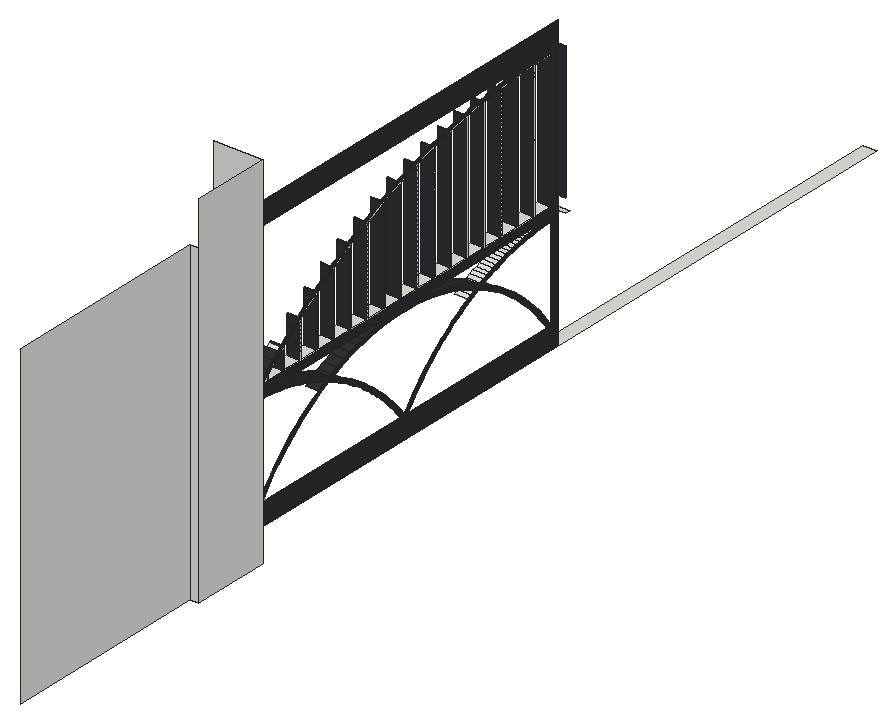
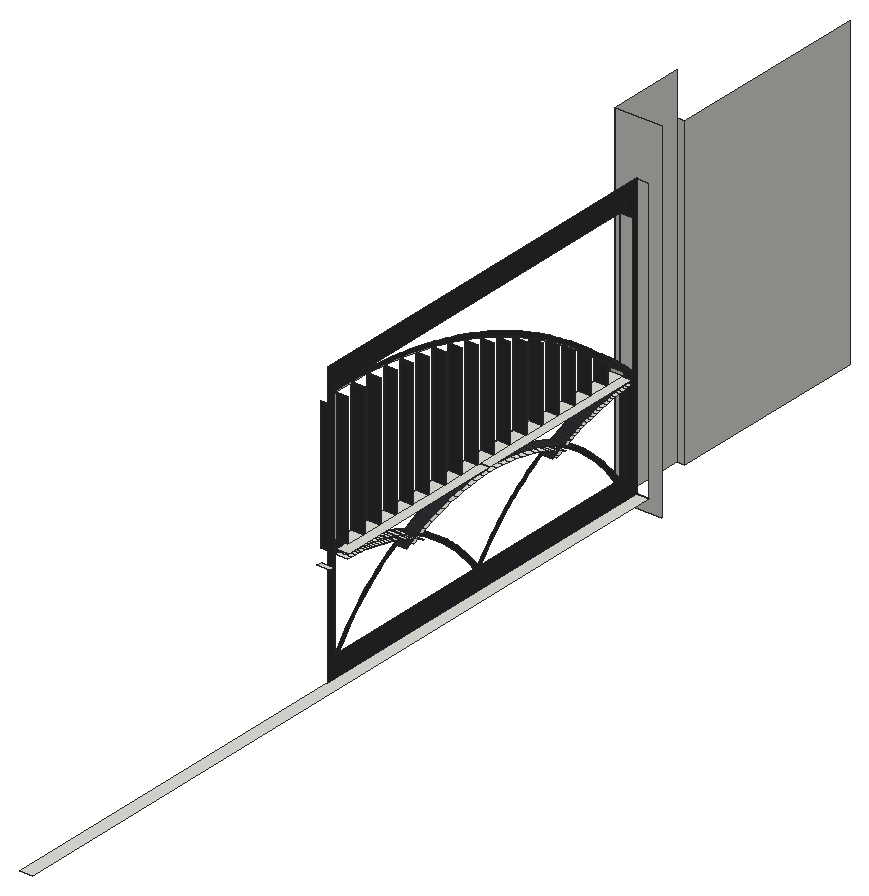
# SketchUp Ruby script. Lengths in inches.
U = 1.inch
M = Sketchup.active_model
def pt(a) = Geom::Point3d.new(a.map { |v| v * U })
def face(e, loops, mat)
  f = e.add_face(loops[0].map { |a| pt(a) })
  loops[1..].each { |l| e.add_face(l.map { |a| pt(a) }).erase! }
  f.material = f.back_material = mat if mat
  f
end
# faces: each face lists its corners as indices into pts; further lists are holes
def faces(e, pts, list, mat = nil) = list.each { |f| face(e, (f[0].is_a?(Array) ? f : [f]).map { |l| l.map { |i| pts[i] } }, mat) }
# xy, xz, yz: faces in a plane at the given z, y or x. An outline is a flat list of corners, or four numbers for a rectangle; further outlines are holes
def ring(l) = l.size == 4 ? [[l[0], l[1]], [l[2], l[1]], [l[2], l[3]], [l[0], l[3]]] : l.each_slice(2).to_a
def flat(e, list, mat, &to3) = list.each { |f| face(e, (f[0].is_a?(Array) ? f : [f]).map { |l| ring(l).map { |u, v| to3.(u, v) } }, mat) }
def xy(e, z, list, mat = nil) = flat(e, list, mat) { |x, y| [x, y, z] }
def xz(e, y, list, mat = nil) = flat(e, list, mat) { |x, z| [x, y, z] }
def yz(e, x, list, mat = nil) = flat(e, list, mat) { |y, z| [x, y, z] }
def lines(e, pts, list) = list.each { |a, b| e.add_line(pt(pts[a]), pt(pts[b])) }
# prism: a flat outline (further loops are holes) pulled along v
def prism(e, loops, v, mat = nil)
  f = face(e, loops, mat); d = Geom::Vector3d.new(v.map { |x| x * U })
  f.pushpull(f.normal.samedirection?(d) ? d.length : -d.length)
end
def box(e, o, s, mat = nil) = prism(e, [[o, [o[0] + s[0], o[1], o[2]], [o[0] + s[0], o[1] + s[1], o[2]], [o[0], o[1] + s[1], o[2]]]], [0, 0, s[2]], mat)
def at(x, y, z, deg = 0) = Geom::Transformation.translation(pt([x, y, z])) * Geom::Transformation.rotation(ORIGIN, Z_AXIS, deg.degrees)
def axes(o, x, y, z) = Geom::Transformation.new([*x, 0, *y, 0, *z, 0, *pt(o).to_a, 1])
def part(name) = M.definitions.add(name)
# library, detail: a bought-in or finely detailed component or shape, given as its bounding box
def library(name, o, s) = part(name).tap { |d| box(d.entities, o, s) }
def detail(e, o, s) = box(e.add_group.entities, o, s)
def put(e, d, t, mat = nil) = e.add_instance(d, t).tap { |i| i.material = mat if mat }
def group(e, t, mat = nil) = e.add_group.tap { |g| g.transformation = t; g.material = mat if mat }.entities
root = M.entities
M.materials.add("ThomThom - Buttons1").color = [48, 49, 53]
xy(root,27,[[474,66,477,246]])
xy(root,54,[[474,71,477,112.5],[474,112.5,477,153.68]])
xy(root,56.1,[[474,73.6875,477,78.22],[474,78.42,477,82.95],[474,83.15,477,87.68],[474,87.88,477,92.41],[474,92.61,477,97.14],
  [474,97.34,477,101.87],[474,102.07,477,106.6],[474,106.8,477,111.33],[474,111.53,477,116.06],[474,116.26,477,120.79],
  [474,120.99,477,125.52],[474,125.72,477,130.25],[474,130.45,477,134.98],[474,135.18,477,139.71],[474,139.91,477,144.44],
  [474,144.64,477,149.17],[474,149.37,477,153.9]])
xz(root,48,[[480,24,482,96]])
xz(root,66,[[[471,24,482,106],[474,27,477,93]]])
xz(root,71,[[474,56,477,88]])
xz(root,73.6875,[[474,56.1,477,56.96]])
xz(root,78.22,[[474,56.1,477,60.79]],"ThomThom - Buttons1")
xz(root,78.42,[[474,56.1,477,60.95]],"ThomThom - Buttons1")
xz(root,82.95,[[474,56.1,477,64.4]],"ThomThom - Buttons1")
xz(root,83.15,[[474,56.1,477,64.55]],"ThomThom - Buttons1")
xz(root,87.68,[[474,56.1,477,67.66]],"ThomThom - Buttons1")
xz(root,87.88,[[474,56.1,477,67.79]],"ThomThom - Buttons1")
xz(root,92.41,[[474,56.1,477,70.59]],"ThomThom - Buttons1")
xz(root,92.61,[[474,56.1,477,70.71]],"ThomThom - Buttons1")
xz(root,97.14,[[474,56.1,477,73.23]],"ThomThom - Buttons1")
xz(root,97.34,[[474,56.1,477,73.33]],"ThomThom - Buttons1")
xz(root,101.87,[[474,56.1,477,75.59]],"ThomThom - Buttons1")
xz(root,102.07,[[474,56.1,477,75.68]],"ThomThom - Buttons1")
xz(root,106.6,[[474,56.1,477,77.7]],"ThomThom - Buttons1")
xz(root,106.8,[[474,56.1,477,77.78]],"ThomThom - Buttons1")
xz(root,111.33,[[474,56.1,477,79.5625]],"ThomThom - Buttons1")
xz(root,111.53,[[474,56.1,477,79.64]],"ThomThom - Buttons1")
xz(root,116.06,[[474,56.1,477,81.2]],"ThomThom - Buttons1")
xz(root,116.26,[[474,56.1,477,81.26]],"ThomThom - Buttons1")
xz(root,120.79,[[474,56.1,477,82.61]],"ThomThom - Buttons1")
xz(root,120.99,[[474,56.1,477,82.67]],"ThomThom - Buttons1")
xz(root,125.52,[[474,56.1,477,83.82]],"ThomThom - Buttons1")
xz(root,125.72,[[474,56.1,477,83.87]],"ThomThom - Buttons1")
xz(root,130.25,[[474,56.1,477,84.82]],"ThomThom - Buttons1")
xz(root,130.45,[[474,56.1,477,84.86]],"ThomThom - Buttons1")
xz(root,134.98,[[474,56.1,477,85.62]],"ThomThom - Buttons1")
xz(root,135.18,[[474,56.1,477,85.65]],"ThomThom - Buttons1")
xz(root,139.71,[[474,56.1,477,86.23]],"ThomThom - Buttons1")
xz(root,139.91,[[474,56.1,477,86.25]],"ThomThom - Buttons1")
xz(root,144.44,[[474,56.1,477,86.64]],"ThomThom - Buttons1")
xz(root,144.64,[[474,56.1,477,86.66]],"ThomThom - Buttons1")
xz(root,149.17,[[474,56.1,477,86.86]],"ThomThom - Buttons1")
xz(root,149.37,[[474,56.1,477,86.87]],"ThomThom - Buttons1")
xz(root,153.9,[[474,56.1,477,86.9]],"ThomThom - Buttons1")
xz(root,158.1,[[474,56.1,477,86.9]],"ThomThom - Buttons1")
yz(root,477,[[112.15,32,112.53,32,112.34,32.25],[72.46,56,73.59,56,73.59,57],[[73.59,56,78.32,56,78.32,61,77.12,60.03,75.73,58.87,74.36,57.69,73.59,57],[73.6875,56.1,73.6875,56.96,74.43,57.62,75.8,58.79,77.18,59.95,78.22,60.79,78.22,56.1]],[[78.32,56,83.05,56,83.05,64.6,82.84,64.45,81.39,63.38,79.95,62.28,78.53,61.17,78.32,61],[78.42,56.1,78.42,60.95,78.59,61.09,80.01,62.21,81.45,63.3,82.9,64.37,82.95,64.4,82.95,56.1]],[[83.05,56,87.78,56,87.78,67.84,87.3,67.53,85.8,66.53,84.3125,65.5,83.05,64.6],[83.15,56.1,83.15,64.55,84.37,65.42,85.86,66.45,87.36,67.45,87.68,67.66,87.68,56.1]],
  [[87.78,56,92.51,56,92.51,70.76,91.9,70.41,90.35,69.47,88.82,68.52,87.78,67.84],[87.88,56.1,87.88,67.79,88.875,68.43,90.41,69.39,91.95,70.32,92.41,70.59,92.41,56.1]],[[92.51,56,97.24,56,97.24,73.39,96.625,73.07,95.04,72.21,93.46,71.32,92.51,70.76],[92.61,56.1,92.61,70.71,93.51,71.23,95.09,72.12,96.67,72.98,97.14,73.23,97.14,56.1]],[[97.24,56,101.97,56,101.97,75.75,101.47,75.51,99.84,74.72,98.23,73.91,97.24,73.39],[97.34,56.1,97.34,73.33,98.27,73.82,99.89,74.63,101.51,75.42,101.87,75.59,101.87,56.1]],[[101.97,56,106.7,56,106.7,77.85,106.42,77.73,104.76,77.02,103.11,76.28,101.97,75.75],[102.07,56.1,102.07,75.68,103.15,76.1875,104.8,76.93,106.45,77.64,106.6,77.7,106.6,56.1]],[[106.7,56,111.43,56,111.43,79.71,109.77,79.08,108.09,78.42,106.7,77.85],[106.8,56.1,106.8,77.78,108.125,78.33,109.81,78.99,111.33,79.5625,111.33,56.1]],
  [[111.43,56,116.16,56,116.16,81.34,114.87,80.92,113.16,80.33,111.46,79.72,111.43,79.71],[111.53,56.1,111.53,79.64,113.2,80.24,114.9,80.82,116.06,81.2,116.06,56.1]],[[116.16,56,120.89,56,120.89,82.75,120.05,82.52,118.32,82.01,116.59,81.48,116.16,81.34],[116.26,56.1,116.26,81.26,116.62,81.38,118.35,81.91,120.08,82.42,120.79,82.61,120.79,56.1]],[[120.89,56,125.62,56,125.62,83.95,125.3,83.875,123.55,83.45,121.8,83,120.89,82.75],[120.99,56.1,120.99,82.67,121.82,82.9,123.57,83.35,125.33,83.78,125.52,83.82,125.52,56.1]],[[125.62,56,130.35,56,130.35,84.94,128.84,84.65,127.07,84.28,125.62,83.95],[125.72,56.1,125.72,83.87,127.09,84.18,128.86,84.55,130.25,84.82,130.25,56.1]],[[130.35,56,135.08,56,135.08,85.74,134.17,85.6,132.39,85.3125,130.61,84.99,130.35,84.94],[130.45,56.1,130.45,84.86,130.63,84.9,132.41,85.21,134.1875,85.51,134.98,85.62,134.98,56.1]],
  [[135.08,56,139.81,56,139.81,86.34,139.55,86.31,137.75,86.11,135.96,85.87,135.08,85.74],[135.18,56.1,135.18,85.65,135.98,85.77,137.77,86.01,139.56,86.22,139.71,86.23,139.71,56.1]],[[139.81,56,144.54,56,144.54,86.75,143.15,86.65,141.35,86.5,139.81,86.34],[139.91,56.1,139.91,86.25,141.36,86.4,143.16,86.55,144.44,86.64,144.44,56.1]],[[144.54,56,149.27,56,149.27,86.97,148.5625,86.95,146.76,86.88,144.95,86.78,144.54,86.75],[144.64,56.1,144.64,86.66,144.96,86.68,146.76,86.78,148.57,86.85,149.17,86.86,149.17,56.1]],[[149.27,56,154,56,154,87,151,87,150.37,86.99,149.27,86.97],[149.37,56.1,149.37,86.87,150.37,86.89,151,86.9,153.9,86.9,153.9,56.1]]])
yz(root,477,[[66,27,156,27,156,30,69,30,69,90,156,90,156,93,66,93],[[69,30,156,90],[71,32,71,88,151,88,152.18,88.01,154,88,154,32]],[71,32,72.22,32,72.93,33,74.1,34.52,75.33,36,76.61,37.42,77.94,38.8,79.33,40.12,80.77,41.38,82.26,42.59,83.79,43.74,85.37,44.83,86.98,45.86,88.64,46.82,90.33,47.72,91.19,48.13,92.39,47.6,92.97,47.31,93.82,46.87,94.66,46.42,95.49,45.95,96.31,45.46,97.12,44.96,97.93,44.45,98.72,43.92,99.51,43.38,100.28,42.82,101.05,42.25,101.8,41.67,102.55,41.07,103.28,40.46,104,39.84,104.71,39.2,105.41,38.55,106.1,37.89,106.78,37.22,107.44,36.53,108.09,35.83,108.73,35.12,109.36,34.4,109.97,33.67,110.51,33,111.3125,32,112.15,32,112.34,32.25,111.95,32.78,111.35,33.55,110.74,34.3,110.12,35.05,109.48,35.78,108.83,36.51,108.17,37.22,107.49,37.92,106.8,38.6,106.1,39.28,105.39,39.94,104.66,40.59,103.93,41.22,103.18,41.85,102.42,42.46,101.65,43.05,100.87,43.63,100.08,44.2,99.28,44.75,98.47,45.29,97.65,45.8125,96.82,46.32,95.99,46.8125,95.14,47.29,94.28,47.75,93.42,48.2,92.55,48.63,92.41,48.7,93.82,49.31,95.6,50,97.42,50.63,99.25,51.18,101.11,51.66,102.98,52.07,104.87,52.4,106.76,52.66,108.67,52.85,110.58,52.96,112.5,53,114.42,52.96,116.33,52.85,118.24,52.66,120.13,52.4,122.02,52.07,123.89,51.66,125.75,51.18,127.58,50.63,129.4,50,131.18,49.31,132.42,48.77,132.27,48.7,132.13,48.63,131.26,48.2,130.4,47.75,129.54,47.29,128.69,46.8125,127.86,46.32,127.03,45.8125,126.21,45.29,125.4,44.75,124.6,44.2,123.81,43.63,123.03,43.05,122.26,42.46,121.5,41.85,120.75,41.22,120.02,40.59,119.29,39.94,118.58,39.28,117.88,38.6,117.19,37.92,116.51,37.22,115.85,36.51,115.2,35.78,114.5625,35.05,113.9375,34.3,113.33,33.55,112.73,32.78,112.34,32.25,112.53,32,113.37,32,114.71,33.67,115.32,34.4,115.95,35.12,116.59,35.83,117.24,36.53,117.9,37.22,118.58,37.89,119.27,38.55,119.97,39.2,120.68,39.84,121.4,40.46,122.13,41.07,122.875,41.67,123.63,42.25,124.4,42.82,125.17,43.38,125.96,43.92,126.75,44.45,127.56,44.96,128.37,45.46,129.19,45.95,130.02,46.42,130.86,46.87,131.71,47.31,133.58,48.24,134.67,47.72,136.36,46.82,138.02,45.86,139.63,44.83,141.21,43.74,142.74,42.59,144.23,41.38,145.67,40.12,147.06,38.8,148.39,37.42,149.67,36,150.9,34.52,152.07,33,152.84,32,154,32,152.87,33.6,151.68,35.15,150.43,36.65,149.125,38.11,147.76,39.51,146.34,40.85,144.875,42.15,143.36,43.38,141.79,44.55,140.1875,45.66,138.54,46.71,136.84,47.69,135.12,48.61,134.72,48.8,136.06,49.27,136.95,49.62,137.85,49.95,138.75,50.26,139.65,50.56,140.57,50.84,141.48,51.1,142.41,51.35,143.33,51.58,144.26,51.79,145.2,51.99,146.13,52.17,147.07,52.33,148.02,52.48,148.96,52.61,149.91,52.72,150.86,52.82,151.8125,52.9,152.76,52.96,154,53.01,154,54,153.68,54,152.71,53.96,151.74,53.89,150.77,53.8125,149.8,53.72,148.84,53.6,147.87,53.47,146.91,53.32,145.95,53.15,145,52.97,144.05,52.77,143.1,52.55,142.16,52.32,141.22,52.07,140.28,51.8,139.35,51.51,138.43,51.21,137.51,50.89,136.6,50.55,135.69,50.2,134.79,49.83,133.9,49.45,133.625,49.33,133.36,49.46,131.5625,50.24,129.74,50.94,127.89,51.58,126.02,52.14,124.125,52.63,122.21,53.05,120.29,53.39,118.35,53.66,116.41,53.85,114.45,53.96,112.5,54,110.55,53.96,108.59,53.85,106.65,53.66,104.71,53.39,102.79,53.05,100.875,52.63,98.98,52.14,97.11,51.58,95.26,50.94,93.4375,50.24,91.64,49.46,91.22,49.25,90.78,49.45,89.89,49.83,88.99,50.2,88.08,50.55,87.17,50.89,86.25,51.21,85.33,51.51,84.4,51.8,83.46,52.07,82.52,52.32,81.58,52.55,80.63,52.77,79.68,52.97,78.73,53.15,77.77,53.32,76.81,53.47,75.84,53.6,74.88,53.72,73.91,53.8125,72.94,53.89,71.97,53.96,71,54,71,53.02,72,52.95,72.87,52.9,73.82,52.82,74.77,52.72,75.72,52.61,76.66,52.48,77.61,52.33,78.55,52.17,79.48,51.99,80.42,51.79,81.35,51.58,82.27,51.35,83.2,51.1,84.11,50.84,85.03,50.56,85.93,50.26,86.83,49.95,87.73,49.62,88.62,49.27,88.84,49.1875,90,48.67,89.88,48.61,88.16,47.69,86.46,46.71,84.8125,45.66,83.21,44.55,81.64,43.38,80.125,42.15,78.66,40.85,77.24,39.51,75.875,38.11,74.57,36.65,73.32,35.15,72.13,33.6],[71,54,154,56],[71,56,72.46,56,73.59,57,74.36,57.69,75.73,58.87,77.12,60.03,78.32,61,78.53,61.17,79.95,62.28,81.39,63.38,82.84,64.45,83.05,64.6,84.3125,65.5,85.8,66.53,87.3,67.53,87.78,67.84,88.82,68.52,90.35,69.47,91.9,70.41,92.51,70.76,93.46,71.32,95.04,72.21,96.625,73.07,97.24,73.39,98.23,73.91,99.84,74.72,101.47,75.51,101.97,75.75,103.11,76.28,104.76,77.02,106.42,77.73,106.7,77.85,108.09,78.42,109.77,79.08,111.43,79.71,111.46,79.72,113.16,80.33,114.87,80.92,116.59,81.48,118.32,82.01,120.05,82.52,120.89,82.75,121.8,83,123.55,83.45,125.3,83.875,125.62,83.95,127.07,84.28,128.84,84.65,130.35,84.94,130.61,84.99,132.39,85.3125,134.17,85.6,135.08,85.74,135.96,85.87,137.75,86.11,139.55,86.31,139.81,86.34,141.35,86.5,143.15,86.65,144.54,86.75,144.95,86.78,146.76,86.88,148.5625,86.95,149.27,86.97,150.37,86.99,151,87,154,87,154,88,151,88,150.35,87.99,148.53,87.95,146.71,87.875,144.89,87.78,143.07,87.65,141.25,87.49,139.44,87.31,137.63,87.1,135.82,86.86,135.08,86.75,134.02,86.59,132.22,86.3,130.43,85.98,130.35,85.96,128.64,85.63,126.85,85.25,125.62,84.97,125.08,84.85,123.3,84.42,121.54,83.96,120.89,83.78,119.78,83.48,118.03,82.97,116.29,82.43,116.16,82.39,114.56,81.87,112.83,81.28,111.43,80.77,111.12,80.66,109.41,80.02,107.71,79.35,106.7,78.93,106.03,78.65,104.35,77.93,102.69,77.1875,101.97,76.85,101.04,76.42,99.4,75.62,97.77,74.8,97.24,74.52,96.16,73.95,94.55,73.08,92.97,72.1875,92.51,71.92,91.39,71.27,89.83,70.33,88.28,69.36,87.78,69.03,86.75,68.37,85.24,67.36,83.74,66.32,83.05,65.83,82.25,65.26,80.79,64.18,79.34,63.08,78.32,62.28,77.9,61.95,76.49,60.8,75.09,59.63,73.71,58.44,73.59,58.34,72.34,57.23]],"ThomThom - Buttons1")
yz(root,480,[[0,24,48,96]])
yz(root,482,[[48,24,66,106]])
p = [[477,92.97,47.31],[477,92.39,47.6],[474,92.39,47.6],[474,92.97,47.31],[477,133.58,48.24],[477,131.71,47.31],
  [474,131.71,47.31],[474,133.58,48.24],[477,91.19,48.13],[474,91.19,48.13],[477,88.16,47.69],[477,89.88,48.61],
  [474,89.88,48.61],[474,88.16,47.69],[477,90.33,47.72],[474,90.33,47.72],[477,134.67,47.72],[474,134.67,47.72],
  [477,135.12,48.61],[477,136.84,47.69],[474,136.84,47.69],[474,135.12,48.61],[477,93.42,48.2],[477,94.28,47.75],
  [474,94.28,47.75],[474,93.42,48.2],[477,130.4,47.75],[477,131.26,48.2],[474,131.26,48.2],[474,130.4,47.75],
  [477,92.55,48.63],[474,92.55,48.63],[477,132.13,48.63],[474,132.13,48.63],[477,90,48.67],[474,90,48.67],
  [477,92.41,48.7],[474,92.41,48.7],[477,132.27,48.7],[474,132.27,48.7],[477,134.72,48.8],[474,134.72,48.8],
  [477,88.84,49.1875],[474,88.84,49.1875],[477,93.82,49.31],[474,93.82,49.31],[477,132.42,48.77],[474,132.42,48.77],
  [477,131.18,49.31],[474,131.18,49.31],[477,136.06,49.27],[474,136.06,49.27],[477,88.62,49.27],[474,88.62,49.27],
  [477,87.73,49.62],[474,87.73,49.62],[477,90.78,49.45],[477,91.22,49.25],[474,91.22,49.25],[474,90.78,49.45],
  [477,91.64,49.46],[474,91.64,49.46],[477,95.6,50],[474,95.6,50],[477,129.4,50],[474,129.4,50],
  [477,133.36,49.46],[477,133.625,49.33],[474,133.625,49.33],[474,133.36,49.46],[477,133.9,49.45],[474,133.9,49.45],
  [477,136.95,49.62],[474,136.95,49.62],[477,89.89,49.83],[474,89.89,49.83],[477,93.4375,50.24],[474,93.4375,50.24],
  [477,131.5625,50.24],[474,131.5625,50.24],[477,134.79,49.83],[474,134.79,49.83],[477,86.83,49.95],[474,86.83,49.95],
  [477,137.85,49.95],[474,137.85,49.95],[477,88.99,50.2],[474,88.99,50.2],[477,135.69,50.2],[474,135.69,50.2],
  [477,85.93,50.26],[474,85.93,50.26],[477,138.75,50.26],[474,138.75,50.26],[477,97.42,50.63],[474,97.42,50.63],
  [477,127.58,50.63],[474,127.58,50.63],[477,88.08,50.55],[474,88.08,50.55],[477,95.26,50.94],[474,95.26,50.94],
  [477,129.74,50.94],[474,129.74,50.94],[477,136.6,50.55],[474,136.6,50.55],[477,85.03,50.56],[474,85.03,50.56],
  [477,139.65,50.56],[474,139.65,50.56],[477,84.11,50.84],[474,84.11,50.84],[477,87.17,50.89],[474,87.17,50.89],
  [477,99.25,51.18],[474,99.25,51.18],[477,125.75,51.18],[474,125.75,51.18],[477,137.51,50.89],[474,137.51,50.89],
  [477,140.57,50.84],[474,140.57,50.84],[477,83.2,51.1],[474,83.2,51.1],[477,141.48,51.1],[474,141.48,51.1],
  [477,86.25,51.21],[474,86.25,51.21],[477,97.11,51.58],[474,97.11,51.58],[477,127.89,51.58],[474,127.89,51.58],
  [477,138.43,51.21],[474,138.43,51.21],[477,82.27,51.35],[474,82.27,51.35],[477,142.41,51.35],[474,142.41,51.35],
  [477,85.33,51.51],[474,85.33,51.51],[477,101.11,51.66],[474,101.11,51.66],[477,123.89,51.66],[474,123.89,51.66],
  [477,139.35,51.51],[474,139.35,51.51],[477,81.35,51.58],[474,81.35,51.58],[477,143.33,51.58],[474,143.33,51.58],
  [477,84.4,51.8],[474,84.4,51.8],[477,140.28,51.8],[474,140.28,51.8],[477,80.42,51.79],[474,80.42,51.79],
  [477,98.98,52.14],[474,98.98,52.14],[477,126.02,52.14],[474,126.02,52.14],[477,144.26,51.79],[474,144.26,51.79],
  [477,102.98,52.07],[474,102.98,52.07],[477,122.02,52.07],[474,122.02,52.07],[477,79.48,51.99],[474,79.48,51.99],
  [477,83.46,52.07],[474,83.46,52.07],[477,141.22,52.07],[474,141.22,52.07],[477,145.2,51.99],[474,145.2,51.99],
  [477,78.55,52.17],[474,78.55,52.17],[477,146.13,52.17],[474,146.13,52.17],[477,82.52,52.32],[474,82.52,52.32],
  [477,100.875,52.63],[474,100.875,52.63],[477,104.87,52.4],[474,104.87,52.4],[477,120.13,52.4],[474,120.13,52.4],
  [477,124.125,52.63],[474,124.125,52.63],[477,142.16,52.32],[474,142.16,52.32],[477,77.61,52.33],[474,77.61,52.33],
  [477,147.07,52.33],[474,147.07,52.33],[477,76.66,52.48],[474,76.66,52.48],[477,81.58,52.55],[474,81.58,52.55],
  [477,143.1,52.55],[474,143.1,52.55],[477,148.02,52.48],[474,148.02,52.48],[477,106.76,52.66],[474,106.76,52.66],
  [477,118.24,52.66],[474,118.24,52.66],[477,75.72,52.61],[474,75.72,52.61],[477,148.96,52.61],[474,148.96,52.61],
  [477,74.77,52.72],[474,74.77,52.72],[477,80.63,52.77],[474,80.63,52.77],[477,102.79,53.05],[474,102.79,53.05],
  [477,122.21,53.05],[474,122.21,53.05],[477,144.05,52.77],[474,144.05,52.77],[477,149.91,52.72],[474,149.91,52.72],
  [477,73.82,52.82],[474,73.82,52.82],[477,108.67,52.85],[474,108.67,52.85],[477,116.33,52.85],[474,116.33,52.85],
  [477,150.86,52.82],[474,150.86,52.82],[477,72.87,52.9],[474,72.87,52.9],[477,79.68,52.97],[474,79.68,52.97],
  [477,145,52.97],[474,145,52.97],[477,151.8125,52.9],[474,151.8125,52.9],[477,72,52.95],[474,72,52.95],
  [477,110.58,52.96],[474,110.58,52.96],[477,114.42,52.96],[474,114.42,52.96],[477,152.76,52.96],[474,152.76,52.96],
  [477,71,53.02],[474,71,53.02],[477,78.73,53.15],[474,78.73,53.15],[477,104.71,53.39],[474,104.71,53.39],
  [477,112.5,53],[474,112.5,53],[477,120.29,53.39],[474,120.29,53.39],[477,145.95,53.15],[474,145.95,53.15],
  [477,154,53.01],[474,154,53.01],[477,159.24,52.96],[477,158,53.01],[474,158,53.01],[474,159.24,52.96],
  [477,77.77,53.32],[474,77.77,53.32],[477,146.91,53.32],[474,146.91,53.32],[477,76.81,53.47],[474,76.81,53.47],
  [477,147.87,53.47],[474,147.87,53.47],[477,106.65,53.66],[474,106.65,53.66],[477,118.35,53.66],[474,118.35,53.66],
  [477,75.84,53.6],[474,75.84,53.6],[477,148.84,53.6],[474,148.84,53.6],[477,74.88,53.72],[474,74.88,53.72],
  [477,149.8,53.72],[474,149.8,53.72],[477,73.91,53.8125],[474,73.91,53.8125],[477,108.59,53.85],[474,108.59,53.85],
  [477,116.41,53.85],[474,116.41,53.85],[477,150.77,53.8125],[474,150.77,53.8125],[477,72.94,53.89],[474,72.94,53.89],
  [477,110.55,53.96],[474,110.55,53.96],[477,114.45,53.96],[474,114.45,53.96],[477,151.74,53.89],[474,151.74,53.89],
  [477,71.97,53.96],[474,71.97,53.96],[477,152.71,53.96],[474,152.71,53.96],[477,71,54],[474,71,54],
  [477,112.5,54],[474,112.5,54],[477,153.68,54],[474,153.68,54],[477,71,56],[477,72.34,57.23],
  [474,72.34,57.23],[474,71,56],[477,74.43,57.62],[477,73.6875,56.96],[474,73.6875,56.96],[474,74.43,57.62],
  [477,73.59,58.34],[474,73.59,58.34],[477,75.8,58.79],[474,75.8,58.79],[477,73.71,58.44],[474,73.71,58.44],
  [477,75.09,59.63],[474,75.09,59.63],[477,77.18,59.95],[474,77.18,59.95],[477,76.49,60.8],[474,76.49,60.8],
  [477,78.22,60.79],[474,78.22,60.79],[477,136.03,49.26]]
faces(root,p,[[0,1,2,3],[4,5,6,7],[1,8,9,2],[8,14,15,9],[16,4,7,17],[26,27,28,29],[27,32,33,28],[32,38,39,33],
  [34,42,43,35],[44,36,37,45],[38,46,47,39],[46,48,49,47],[50,40,41,51],[42,52,53,43],[52,54,55,53],[62,44,45,63],
  [48,64,65,49],[67,70,71,68],[72,50,51,73],[70,80,81,71],[54,82,83,55],[84,72,73,85],[80,88,89,81],[82,90,91,83],
  [92,84,85,93],[94,62,63,95],[64,96,97,65],[88,104,105,89],[90,106,107,91],[108,92,93,109],[106,110,111,107],[114,94,95,115],
  [96,116,117,97],[104,118,119,105],[120,108,109,121],[110,122,123,111],[124,120,121,125],[118,132,133,119],[122,134,135,123],[136,124,125,137],
  [140,114,115,141],[116,142,143,117],[132,144,145,133],[134,146,147,135],[148,136,137,149],[144,152,153,145],[146,154,155,147],[160,148,149,161],
  [162,140,141,163],[142,164,165,143],[154,166,167,155],[152,170,171,153],[172,160,161,173],[166,174,175,167],[176,172,173,177],[182,162,163,183],
  [164,184,185,165],[170,188,189,171],[174,190,191,175],[192,176,177,193],[190,194,195,191],[188,198,199,189],[200,192,193,201],[202,182,183,203],
  [184,204,205,185],[194,206,207,195],[208,200,201,209],[206,210,211,207],[198,218,219,199],[220,208,209,221],[210,222,223,211],[224,202,203,225],
  [204,226,227,205],[228,220,221,229],[222,230,231,223],[218,234,235,219],[236,228,229,237],[230,238,239,231],[240,224,225,241],[226,242,243,227],
  [244,236,237,245],[238,246,247,239],[252,240,241,253],[242,252,253,243],[234,256,257,235],[258,244,245,259],[260,261,262,263],[256,266,267,257],
  [266,270,271,267],[270,278,279,271],[278,282,283,279],[282,290,291,283],[290,298,299,291],[298,302,303,299],[302,308,309,303],[314,315,316,317],
  [320,314,317,321],[326,320,321,327],[330,326,327,331]])
faces(root,p,[[10,11,12,13],[18,19,20,21],[22,23,24,25],[30,22,25,31],[11,34,35,12],[36,30,31,37],[40,18,21,41],[56,57,58,59],
  [57,60,61,58],[66,67,68,69],[74,56,59,75],[60,76,77,61],[78,66,69,79],[86,74,75,87],[98,86,87,99],[76,100,101,77],
  [102,78,79,103],[112,98,99,113],[126,112,113,127],[100,128,129,101],[130,102,103,131],[138,126,127,139],[150,138,139,151],[128,156,157,129],
  [158,130,131,159],[168,150,151,169],[178,168,169,179],[156,180,181,157],[186,158,159,187],[196,178,179,197],[212,196,197,213],[180,214,215,181],
  [216,186,187,217],[232,212,213,233],[248,232,233,249],[214,250,251,215],[254,216,217,255],[264,248,249,265],[268,264,265,269],[250,272,273,251],
  [274,254,255,275],[276,268,269,277],[280,276,277,281],[284,280,281,285],[272,286,287,273],[288,274,275,289],[292,284,285,293],[286,294,295,287],
  [296,288,289,297],[300,292,293,301],[304,300,301,305],[294,306,307,295],[306,296,297,307],[310,311,312,313],[311,318,319,312],[318,322,323,319],
  [322,324,325,323],[324,328,329,325]],"ThomThom - Buttons1")
lines(root,p,[[50,332]])
